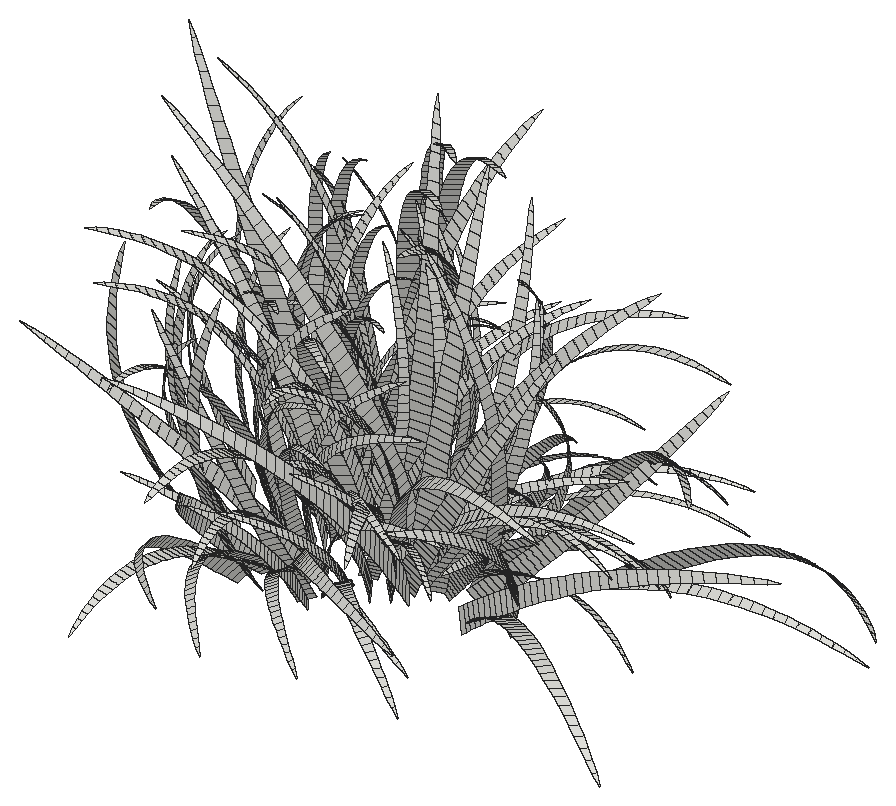
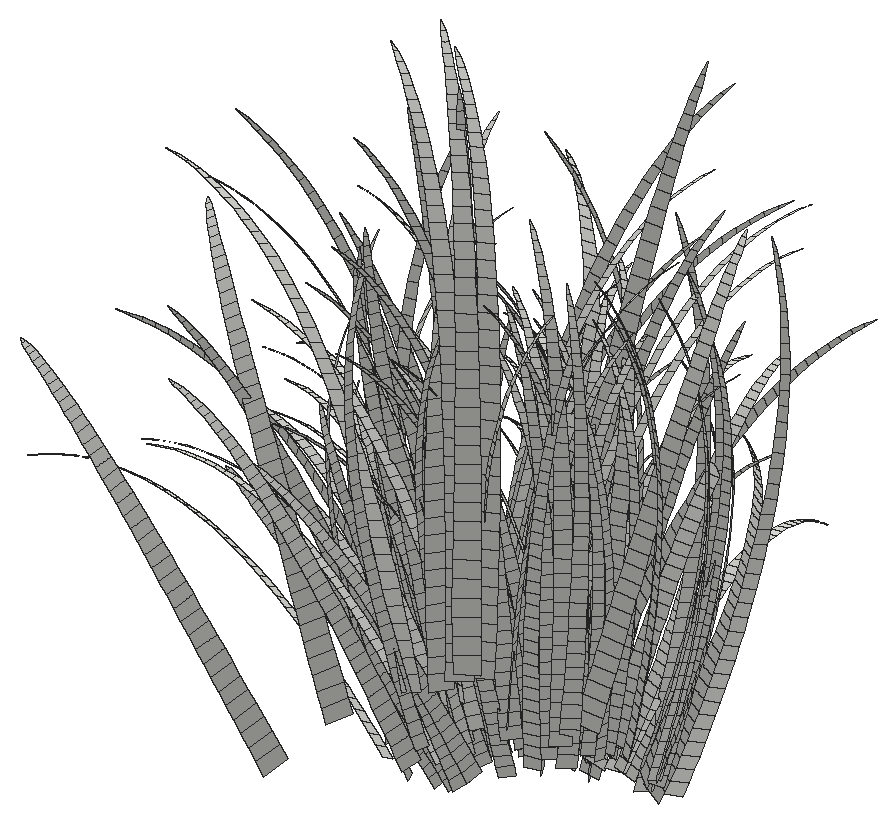
# SketchUp Ruby script. Lengths in inches.
U = 1.inch
M = Sketchup.active_model
def pt(a) = Geom::Point3d.new(a.map { |v| v * U })
def face(e, loops, mat)
  f = e.add_face(loops[0].map { |a| pt(a) })
  loops[1..].each { |l| e.add_face(l.map { |a| pt(a) }).erase! }
  f.material = f.back_material = mat if mat
  f
end
# faces: each face lists its corners as indices into pts; further lists are holes
def faces(e, pts, list, mat = nil) = list.each { |f| face(e, (f[0].is_a?(Array) ? f : [f]).map { |l| l.map { |i| pts[i] } }, mat) }
# xy, xz, yz: faces in a plane at the given z, y or x. An outline is a flat list of corners, or four numbers for a rectangle; further outlines are holes
def ring(l) = l.size == 4 ? [[l[0], l[1]], [l[2], l[1]], [l[2], l[3]], [l[0], l[3]]] : l.each_slice(2).to_a
def flat(e, list, mat, &to3) = list.each { |f| face(e, (f[0].is_a?(Array) ? f : [f]).map { |l| ring(l).map { |u, v| to3.(u, v) } }, mat) }
def xy(e, z, list, mat = nil) = flat(e, list, mat) { |x, y| [x, y, z] }
def xz(e, y, list, mat = nil) = flat(e, list, mat) { |x, z| [x, y, z] }
def yz(e, x, list, mat = nil) = flat(e, list, mat) { |y, z| [x, y, z] }
def lines(e, pts, list) = list.each { |a, b| e.add_line(pt(pts[a]), pt(pts[b])) }
# prism: a flat outline (further loops are holes) pulled along v
def prism(e, loops, v, mat = nil)
  f = face(e, loops, mat); d = Geom::Vector3d.new(v.map { |x| x * U })
  f.pushpull(f.normal.samedirection?(d) ? d.length : -d.length)
end
def box(e, o, s, mat = nil) = prism(e, [[o, [o[0] + s[0], o[1], o[2]], [o[0] + s[0], o[1] + s[1], o[2]], [o[0], o[1] + s[1], o[2]]]], [0, 0, s[2]], mat)
def at(x, y, z, deg = 0) = Geom::Transformation.translation(pt([x, y, z])) * Geom::Transformation.rotation(ORIGIN, Z_AXIS, deg.degrees)
def axes(o, x, y, z) = Geom::Transformation.new([*x, 0, *y, 0, *z, 0, *pt(o).to_a, 1])
def part(name) = M.definitions.add(name)
# library, detail: a bought-in or finely detailed component or shape, given as its bounding box
def library(name, o, s) = part(name).tap { |d| box(d.entities, o, s) }
def detail(e, o, s) = box(e.add_group.entities, o, s)
def put(e, d, t, mat = nil) = e.add_instance(d, t).tap { |i| i.material = mat if mat }
def group(e, t, mat = nil) = e.add_group.tap { |g| g.transformation = t; g.material = mat if mat }.entities
root = M.entities
c1 = part("fur_instance\#8")
p = [[-0.25,1.49,0.03],[0.25,-1.49,-0.03],[0.44,-1.47,1.51],[-0.05,1.47,1.57],[0.65,-1.44,3.05],[0.16,1.45,3.11],
  [0.86,-1.42,4.59],[0.38,1.44,4.65],[1.1,-1.39,6.13],[0.62,1.43,6.18],[1.34,-1.35,7.66],[0.875,1.42,7.72],
  [1.6,-1.32,9.19],[1.14,1.41,9.25],[1.88,-1.28,10.72],[1.43,1.41,10.78],[2.18,-1.24,12.25],[1.73,1.41,12.3],
  [2.49,-1.19,13.77],[2.05,1.41,13.82],[2.83,-1.15,15.29],[2.4,1.41,15.34],[3.18,-1.09,16.8],[2.76,1.42,16.85],
  [3.56,-1.03,18.31],[3.14,1.43,18.35],[3.96,-0.97,19.81],[3.55,1.44,19.85],[4.38,-0.91,21.3],[3.99,1.46,21.35],
  [4.84,-0.83,22.78],[4.45,1.48,22.83],[5.32,-0.76,24.26],[4.93,1.51,24.31],[5.82,-0.67,25.73],[5.45,1.54,25.77],
  [6.36,-0.59,27.18],[6,1.57,27.23],[6.93,-0.49,28.625],[6.58,1.61,28.67],[7.54,-0.39,30.05],[7.19,1.66,30.1],
  [8.18,-0.28,31.47],[7.84,1.71,31.51],[8.85,-0.16,32.86],[8.53,1.77,32.9],[9.57,-0.04,34.24],[9.25,1.83,34.27],
  [10.32,0.09,35.59],[10.02,1.9,35.625],[11.12,0.23,36.92],[10.82,1.97,36.95],[11.95,0.38,38.22],[11.67,2.06,38.25],
  [12.84,0.54,39.49],[12.57,2.14,39.52],[13.76,0.71,40.73],[13.51,2.24,40.76],[14.73,0.89,41.93],[14.49,2.34,41.95],
  [15.75,1.08,43.09],[15.52,2.45,43.11],[16.82,1.28,44.2],[16.6,2.5625,44.23],[17.93,1.5,45.27],[17.73,2.68,45.29],
  [19.08,1.73,46.28],[18.9,2.81,46.3],[20.29,1.97,47.24],[20.125,2.93,47.26],[21.53,2.22,48.13],[21.39,3.0625,48.15],
  [22.82,2.5,48.96],[22.7,3.1875,48.98],[24.14,2.8125,49.72],[24.06,3.3,49.73],[25.48,3.27,50.41]]
faces(c1.entities,p,[[0,1,2,3],[3,2,4,5],[5,4,6,7],[7,6,8,9],[9,8,10,11],[11,10,12,13],[13,12,14,15],[15,14,16,17],
  [17,16,18,19],[19,18,20,21],[21,20,22,23],[23,22,24,25],[25,24,26,27],[27,26,28,29],[29,28,30,31],[31,30,32,33],
  [33,32,34,35],[35,34,36,37],[37,36,38,39],[39,38,40,41],[41,40,42,43],[43,42,44,45],[45,44,46,47],[47,46,48,49],
  [49,48,50,51],[51,50,52,53],[53,52,54,55],[55,54,56,57],[57,56,58,59],[59,58,60,61],[61,60,62,63],[63,62,64,65],
  [65,64,66,67],[67,66,68,69],[69,68,70,71],[71,70,72,73],[73,72,74,75],[75,74,76]])
put(root,c1,axes([297.34,24.49,10.07],[0.22754,0.09548,0.30287],[-0.3741,0.10321,0.18489],[-0.01658,-0.28689,0.27555]))
put(root,c1,axes([298.36,29.48,15.33],[0.08571,-0.27266,-0.13744],[0.42739,0.02102,0.03088],[-0.01459,-0.16231,0.42441]))
put(root,c1,axes([298.25,24.62,10.32],[0.14483,0.12085,0.20815],[-0.30882,0.08881,0.09603],[-0.01291,-0.19862,0.26445]))
put(root,c1,axes([297.38,27.93,13.53],[0.30966,0.098,0.10011],[-0.20983,0.22175,0.06913],[-0.05457,-0.13112,0.36799]))
put(root,c1,axes([297.55,26.52,12.34],[0.32914,-0.02019,0.08794],[-0.06155,0.19695,0.14966],[-0.07419,-0.15278,0.30582]))
put(root,c1,axes([302.33,24.8,10.55],[-0.40749,-0.00335,0.18025],[-0.12021,-0.15441,-0.30655],[0.11437,-0.28118,0.27754]))
put(root,c1,axes([299.27,26.41,12.88],[-0.00998,-0.21329,-0.19726],[0.39469,-0.01957,-0.03476],[0.02221,-0.19303,0.35251]))
put(root,c1,axes([297.15,25.85,11.82],[0.33918,0.02077,0.08926],[-0.11622,0.19982,0.16012],[-0.0464,-0.17067,0.32217]))
put(root,c1,axes([302.64,29.66,13.99],[-0.38125,-0.04643,0.1073],[0.06668,-0.27303,-0.05684],[0.10363,-0.09301,0.39245]))
put(root,c1,axes([302.09,25.9375,11.41],[-0.30784,-0.04638,0.08341],[0.04021,-0.18889,-0.13984],[0.09826,-0.13618,0.29147]))
put(root,c1,axes([297.93,24.99,10.86],[0.34312,-0.02724,0.07631],[-0.06105,0.16155,0.2245],[-0.05704,-0.19865,0.27364]))
put(root,c1,axes([298.34,24.67,10.57],[0.25415,0.10614,0.20022],[-0.29634,0.1349,0.16955],[-0.01477,-0.22734,0.30268]))
put(root,c1,axes([302.43,27.59,14.25],[-0.34392,-0.19747,-0.05942],[0.31246,-0.1879,-0.23256],[0.10907,-0.21637,0.42646]))
put(root,c1,axes([298.55,30.67,13.78],[0.22131,-0.22629,0.02615],[0.29382,0.13921,-0.0109],[-0.01591,-0.03849,0.37643]))
put(root,c1,axes([300.79,24.4,10.07],[-0.08897,-0.12733,-0.31327],[0.39814,-0.02359,-0.11091],[0.04663,-0.26995,0.25847]))
put(root,c1,axes([301.35,29.07,12.71],[-0.18067,-0.19345,0.07522],[0.26975,-0.14432,-0.061],[0.08262,-0.03764,0.32955]))
put(root,c1,axes([302.4375,26.68,13.18],[-0.30501,-0.19584,-0.06885],[0.3125,-0.16513,-0.21481],[0.1025,-0.20334,0.40077]))
put(root,c1,axes([300.66,30.47,12.875],[-0.05382,-0.24378,0.08465],[0.33677,-0.06068,-0.04502],[0.04922,-0.00382,0.34004]))
put(root,c1,axes([298.89,26.04,12.12],[0.26522,0.09384,0.11083],[-0.21458,0.15991,0.13303],[-0.0124,-0.16608,0.30419]))
put(root,c1,axes([302.32,24.36,9.24],[-0.2996,-0.07248,0.07639],[0.02633,-0.11445,-0.25289],[0.12958,-0.19663,0.20724]))
put(root,c1,axes([302.84,26.03,12.1],[-0.30808,0.0964,0.26106],[-0.2636,-0.1875,-0.11584],[0.13613,-0.2298,0.33276]))
put(root,c1,axes([302.32,24.34,9.32],[-0.1838,0.08779,0.29069],[-0.31205,-0.09811,-0.08599],[0.09749,-0.23969,0.23659]))
put(root,c1,axes([298.55,28.32,13.11],[0.33703,-0.0606,0.00869],[0.04934,0.22775,0.04178],[-0.02278,-0.08013,0.34741]))
put(root,c1,axes([301.15,28.07,12.85],[-0.08647,-0.22321,-0.0256],[0.3195,-0.05984,-0.10171],[0.08204,-0.09177,0.33353]))
put(root,c1,axes([298.93,24.11,9.43],[0.31431,-0.11382,-0.22646],[0.27893,0.07249,0.25434],[-0.01591,-0.27534,0.26445]))
put(root,c1,axes([299.05,27.16,12.77],[0.30618,-0.11178,-0.04367],[0.14225,0.17991,0.09998],[-0.0113,-0.12571,0.32871]))
put(root,c1,axes([302.84,28.1,12.3],[-0.3018,-0.05533,0.14889],[0.04839,-0.22497,-0.0736],[0.14879,-0.08814,0.30643]))
put(root,c1,axes([298.8,28.85,13.53],[0.33228,-0.11223,-0.01481],[0.12989,0.21816,0.04248],[-0.01045,-0.08682,0.36317]))
put(root,c1,axes([298.86,30.74,14.82],[0.2513,-0.23591,-0.02705],[0.31438,0.16202,-0.0286],[0.02842,-0.06817,0.4118]))
put(root,c1,axes([303.34,26.51,13.1875],[-0.20765,0.20524,0.34836],[-0.46933,-0.12275,-0.04529],[0.10847,-0.29849,0.40724]))
put(root,c1,axes([299.4375,24.06,9.36],[0.23528,0.12192,0.28082],[-0.37572,0.07027,0.22703],[0.05067,-0.29334,0.28087]))
put(root,c1,axes([302.89,29.79,12.49],[-0.26364,-0.1277,0.16127],[0.17439,-0.21809,-0.03735],[0.14552,-0.02258,0.31606]))
put(root,c1,axes([299.78,27.4375,13.63],[0.21857,-0.21363,-0.1219],[0.32632,0.12674,0.03328],[0.03098,-0.14429,0.38367]))
put(root,c1,axes([302.0625,26.01,12.41],[-0.08548,-0.19985,-0.26017],[0.42158,-0.01554,-0.13787],[0.09092,-0.25018,0.34134]))
put(root,c1,axes([299.15,24.38,10.15],[0.39204,-0.05893,-0.06456],[0.07903,0.1141,0.3176],[-0.01514,-0.26203,0.25167]))
put(root,c1,axes([300.34,27.34,13.09],[0.20316,0.18695,0.05206],[-0.29596,0.1361,0.10285],[0.04697,-0.12733,0.35285]))
put(root,c1,axes([300.29,29.89,13.24],[0.241,-0.19394,-0.00595],[0.25165,0.15803,-0.0286],[0.01565,-0.04576,0.35642]))
put(root,c1,axes([300.23,24.37,10.06],[0.20909,-0.10864,-0.30363],[0.35015,0.0704,0.13483],[0.04661,-0.26986,0.25839]))
put(root,c1,axes([302.13,24.96,10.65],[0.0034,-0.17259,-0.2459],[0.3736,0.02284,-0.07022],[0.07897,-0.21729,0.29647]))
put(root,c1,axes([304.83,28.53,14.14],[-0.33019,-0.21589,-0.02043],[0.30998,-0.1841,-0.23665],[0.14334,-0.19866,0.4252]))
put(root,c1,axes([306.23,27.17,12.88],[-0.44601,0.0603,0.27836],[-0.22496,-0.25265,-0.21525],[0.16772,-0.28312,0.40997]))
put(root,c1,axes([300.14,25.48,11.52],[0.31524,-0.06334,-0.07199],[0.09612,0.1672,0.15091],[0.01854,-0.16113,0.29426]))
put(root,c1,axes([305.13,26.27,11.21],[-0.38378,-0.04877,0.18024],[-0.02944,-0.22334,-0.21648],[0.17648,-0.20752,0.33035]))
put(root,c1,axes([301.71,27.32,12.9],[0.09016,-0.23072,-0.1049],[0.34864,0.05757,-0.04796],[0.06396,-0.12072,0.35681]))
put(root,c1,axes([300.71,28.48,12.82],[0.28641,-0.13175,-0.03296],[0.16621,0.19382,-0.00842],[0.02384,-0.06063,0.3387]))
put(root,c1,axes([304.25,25.28,9.26],[-0.26262,-0.12182,0.05251],[0.09128,-0.10048,-0.25575],[0.16729,-0.17618,0.20619]))
put(root,c1,axes([304.83,25.73,9.93],[-0.30829,-0.09539,0.14082],[0.00903,-0.14692,-0.25308],[0.18557,-0.19544,0.22873]))
put(root,c1,axes([302.31,30.2,11.78],[0.03803,-0.23615,0.09237],[0.30529,0.00187,-0.1209],[0.10385,0.01684,0.29612]))
put(root,c1,axes([303.54,26.1875,10.96],[-0.17541,-0.18465,-0.02445],[0.23008,-0.0678,-0.21965],[0.16634,-0.14325,0.26122]))
put(root,c1,axes([301.04,25.375,11.33],[0.25986,-0.11185,-0.13998],[0.20362,0.14616,0.09388],[0.04858,-0.15915,0.29774]))
put(root,c1,axes([300.67,28.46,13.55],[0.22798,-0.18767,-0.11254],[0.27671,0.15509,-0.02037],[0.07789,-0.11087,0.35837]))
put(root,c1,axes([306.9,25.87,10.72],[-0.48988,-0.11693,0.12815],[0.03908,-0.18796,-0.41221],[0.21173,-0.3213,0.33863]))
put(root,c1,axes([304.08,26.78,11.13],[-0.20056,0.10644,0.21815],[-0.1976,-0.18803,0.05052],[0.19039,-0.12136,0.26701]))
put(root,c1,axes([303.36,27.03,12.83],[-0.04495,-0.24966,-0.14848],[0.39596,-0.00054,-0.1471],[0.12613,-0.17481,0.37414]))
put(root,c1,axes([300.875,28.02,12.78],[0.31334,0.05722,-0.07403],[-0.08122,0.21863,0.071],[0.08023,-0.08975,0.32618]))
put(root,c1,axes([304.8,27.75,10.98],[-0.23233,0.07819,0.21635],[-0.13938,-0.21462,0.04879],[0.20297,-0.09356,0.26698]))
put(root,c1,axes([302.16,30.1,13.69],[0.15425,-0.25107,-0.03735],[0.33478,0.10551,-0.10575],[0.09996,-0.05813,0.37518]))
put(root,c1,axes([304.91,27.45,12.12],[-0.25388,-0.20378,0.01616],[0.23529,-0.11773,-0.26393],[0.19902,-0.17138,0.31253]))
put(root,c1,axes([301.81,24.55,10.08],[0.19971,-0.08632,-0.29459],[0.31288,0.10372,0.09875],[0.09992,-0.24566,0.24248]))
put(root,c1,axes([305.41,29.01,11.21],[-0.27508,0.01899,0.22955],[-0.04819,-0.2486,0.02313],[0.21789,-0.06738,0.28047]))
put(root,c1,axes([301.65,28.92,12.46],[0.28163,-0.12087,-0.06722],[0.14848,0.20348,-0.06709],[0.08102,-0.03691,0.32316]))
put(root,c1,axes([300.74,25.01,11.39],[0.45568,0.06765,0.06956],[-0.16773,0.20168,0.31955],[0.04218,-0.28469,0.37786]))
put(root,c1,axes([301.56,25.46,11.47],[0.33477,0.08293,0.02574],[-0.13812,0.14697,0.24654],[0.07654,-0.21062,0.28736]))
put(root,c1,axes([301.31,28.87,13.17],[0.30114,-0.11966,-0.09813],[0.15874,0.2176,-0.03834],[0.09385,-0.06803,0.34638]))
put(root,c1,axes([305.74,28.81,11.7],[-0.28867,0.02967,0.24792],[-0.09166,-0.25361,-0.00275],[0.22689,-0.10459,0.29846]))
put(root,c1,axes([305.46,26.23,9.98],[-0.26784,-0.15803,0.10336],[0.1003,-0.12666,-0.27197],[0.22305,-0.17007,0.23161]))
put(root,c1,axes([302.53,28.71,12.53],[0.22312,-0.17996,-0.07706],[0.24279,0.15961,-0.06691],[0.09091,-0.0659,0.33552]))
put(root,c1,axes([302.11,27.35,14.32],[0.30189,-0.2143,-0.23607],[0.3879,0.17076,0.0851],[0.07233,-0.23695,0.44329]))
put(root,c1,axes([306.3,29.18,11.54],[-0.3066,-0.07009,0.23185],[0.02539,-0.24972,-0.09835],[0.23047,-0.10624,0.30316]))
put(root,c1,axes([302.74,27.47,12.35],[0.21694,0.18488,-0.0402],[-0.23457,0.13588,0.16772],[0.14294,-0.11176,0.31472]))
put(root,c1,axes([306.73,27.34,10.91],[-0.20769,0.14499,0.26631],[-0.28732,-0.19256,0.04919],[0.20383,-0.17553,0.32009]))
put(root,c1,axes([305.49,27.83,13.38],[-0.08102,0.22851,0.2885],[-0.42602,-0.11882,0.13225],[0.19883,-0.2338,0.37219]))
put(root,c1,axes([301.94,25.29,11.29],[0.40091,0.03016,-0.06734],[-0.01586,0.18451,0.26625],[0.0848,-0.23335,0.31837]))
put(root,c1,axes([302.89,32.5,17.82],[0.25572,-0.30691,-0.1555],[0.45234,0.17411,-0.05741],[0.11289,-0.16068,0.51939]))
put(root,c1,axes([303.53,28.55,14.42],[0.21342,0.25446,0.08921],[-0.38491,0.1062,0.2129],[0.1393,-0.19307,0.41321]))
put(root,c1,axes([303.13,24.86,9.67],[0.22226,-0.03579,-0.23917],[0.20428,0.13118,0.1145],[0.13006,-0.19737,0.20802]))
put(root,c1,axes([302.86,26.07,11.88],[0.25415,-0.10802,-0.25116],[0.27378,0.16143,0.07847],[0.12542,-0.21172,0.30658]))
put(root,c1,axes([305.11,31.45,15.75],[-0.0769,-0.31872,-0.07944],[0.43795,-0.01955,-0.2265],[0.19894,-0.15553,0.43799]))
put(root,c1,axes([303.3,30.9375,16.79],[0.29435,-0.27412,-0.16204],[0.41262,0.19204,-0.0101],[0.09002,-0.16992,0.50222]))
put(root,c1,axes([302.8,24.9,10.11],[0.31893,0.00084,-0.14381],[0.07397,0.17023,0.18028],[0.10993,-0.18556,0.2687]))
put(root,c1,axes([303.4375,27.83,13.15],[0.22284,0.22267,0.01676],[-0.30608,0.12329,0.20104],[0.14725,-0.15151,0.36439]))
put(root,c1,axes([304.81,26.24,11.52],[0.02363,-0.22016,-0.24514],[0.39411,0.08072,-0.15296],[0.18102,-0.21286,0.33886]))
put(root,c1,axes([304.35,26.14,10.36],[0.11227,-0.15154,-0.20337],[0.26794,0.12668,-0.08881],[0.16703,-0.14384,0.2623]))
put(root,c1,axes([303.07,32.69,17.52],[0.32353,-0.26537,-0.15942],[0.39128,0.2201,-0.02856],[0.1103,-0.157,0.50748]))
put(root,c1,axes([306.99,28.03,11.25],[-0.12843,0.20843,0.21843],[-0.31581,-0.15815,0.16065],[0.23054,-0.14695,0.32332]))
put(root,c1,axes([306.27,31.36,12.34],[-0.13308,-0.26326,0.14802],[0.2903,-0.12144,-0.21379],[0.24345,-0.04095,0.31921]))
put(root,c1,axes([302.52,24.75,10.52],[0.40095,-0.04465,-0.28976],[0.25669,0.16722,0.27357],[0.12816,-0.31508,0.31101]))
put(root,c1,axes([303.85,24.95,10.14],[0.21212,-0.09265,-0.34742],[0.34111,0.15542,0.06154],[0.17306,-0.26262,0.27679]))
put(root,c1,axes([304.53,27.53,12.17],[0.27009,0.18151,-0.02583],[-0.2385,0.16041,0.19025],[0.14014,-0.14419,0.34679]))
put(root,c1,axes([305.1,30.01,10.22],[0.09946,-0.22813,0.00742],[0.24835,0.06793,-0.21012],[0.1872,-0.00489,0.26052]))
put(root,c1,axes([306.85,26.9,11.58],[-0.00683,0.24532,0.26139],[-0.4333,-0.07786,0.1796],[0.19869,-0.23364,0.37193]))
put(root,c1,axes([305.04,28.56,10.66],[0.10211,-0.20387,-0.09855],[0.23938,0.11146,-0.19109],[0.20305,-0.06279,0.26137]))
put(root,c1,axes([306.16,28.95,9.54],[-0.06535,-0.22674,0.13107],[0.20945,-0.07623,-0.22504],[0.24597,-0.02324,0.21537]))
put(root,c1,axes([306.87,27.41,10.26],[-0.11302,0.153,0.26635],[-0.25481,-0.18419,0.15446],[0.26582,-0.14677,0.2473]))
put(root,c1,axes([307.28,27.4,10.09],[-0.13627,0.14133,0.28477],[-0.25117,-0.20069,0.13612],[0.2725,-0.15046,0.25352]))
put(root,c1,axes([304.38,29.98,10.89],[0.23395,-0.13822,-0.12541],[0.13453,0.19634,-0.17104],[0.18884,-0.00494,0.2628]))
put(root,c1,axes([309.19,28.14,11.03],[-0.30608,0.01652,0.36552],[-0.2093,-0.26205,-0.09314],[0.28918,-0.22048,0.30027]))
put(root,c1,axes([304.77,26.93,10.57],[0.25146,0.13747,-0.12144],[-0.11784,0.16285,0.18448],[0.18778,-0.1197,0.26336]))
put(root,c1,axes([307.41,27.625,10.17],[-0.13638,-0.24622,-0.04178],[0.25232,-0.00872,-0.31404],[0.27351,-0.15102,0.25446]))
put(root,c1,axes([307.96,30.11,9.72],[-0.18802,-0.2009,0.2136],[0.15844,-0.17448,-0.20851],[0.28488,-0.06696,0.24446]))
put(root,c1,axes([306.29,26.3,10.49],[0.15586,0.20567,0.19062],[-0.32905,-0.02152,0.28384],[0.21907,-0.23072,0.27002]))
put(root,c1,axes([305.04,28.98,12.72],[0.33777,-0.06805,-0.19427],[0.11791,0.26248,-0.00695],[0.17416,-0.10316,0.35867]))
put(root,c1,axes([305.88,29.36,9.75],[0.12899,-0.19626,-0.10232],[0.17724,0.13637,-0.23923],[0.24574,-0.02322,0.21517]))
put(root,c1,axes([305.42,27.18,10.76],[0.29043,0.0064,-0.22579],[0.06951,0.22909,0.0737],[0.20194,-0.12872,0.28321]))
put(root,c1,axes([305.96,28.06,11.31],[0.24712,-0.0965,-0.24934],[0.19671,0.22236,-0.03054],[0.21358,-0.13615,0.29954]))
put(root,c1,axes([305.7,26.87,10.97],[0.33871,0.04215,-0.20809],[0.0397,0.228,0.15673],[0.19608,-0.16885,0.30791]))
put(root,c1,axes([310.91,27.67,9.69],[-0.32027,-0.26261,0.03115],[0.24097,-0.10763,-0.40652],[0.31258,-0.23832,0.32457]))
put(root,c1,axes([306.65,29.41,9.66],[0.13998,-0.20119,-0.1139],[0.18152,0.14824,-0.24709],[0.25697,-0.02428,0.225]))
put(root,c1,axes([305.51,29.47,14.17],[0.42752,0.07803,-0.15016],[-0.06383,0.27992,0.17466],[0.16812,-0.17298,0.41603]))
put(root,c1,axes([305.98,29.04,11.375],[0.28212,0.09572,-0.22762],[-0.08022,0.24373,0.08309],[0.22884,-0.07077,0.29456]))
put(root,c1,axes([306.72,28.14,10.05],[0.14119,-0.14163,-0.23922],[0.19799,0.1965,-0.1586],[0.26602,-0.10193,0.23276]))
put(root,c1,axes([305.74,26.48,12.09],[0.42799,-0.0644,-0.27533],[0.2288,0.24399,0.20262],[0.16294,-0.27505,0.39829]))
put(root,c1,axes([306.82,28.16,10.57],[0.24831,-0.10238,-0.23706],[0.17169,0.23302,-0.06981],[0.22616,-0.10425,0.29749]))
put(root,c1,axes([306.53,29.74,10.82],[0.28927,0.00402,-0.23977],[0.02368,0.25909,-0.00208],[0.22645,-0.07003,0.29149]))
put(root,c1,axes([307.02,31.21,11.13],[0.23822,-0.17838,-0.16309],[0.19592,0.21585,-0.19099],[0.23514,-0.03955,0.30831]))
put(root,c1,axes([307.17,27.27,12.13],[0.32533,0.2365,0.05188],[-0.31811,0.13076,0.32893],[0.20862,-0.24531,0.39052]))
put(root,c1,axes([308.75,28.38,9.72],[0.09146,0.2529,0.10201],[-0.28326,-0.03766,0.31256],[0.28385,-0.15672,0.26408]))
put(root,c1,axes([307.4375,30.66,14.51],[0.41841,-0.08805,-0.24207],[0.17069,0.31234,0.03012],[0.20217,-0.15807,0.44512]))
put(root,c1,axes([310.07,27,9.6875],[0.214,-0.12431,-0.41458],[0.3864,0.21791,-0.01296],[0.26577,-0.2799,0.32758]))
put(root,c1,axes([310.85,31.57,12.3125],[0.10249,-0.29776,-0.17699],[0.37955,0.14559,-0.26879],[0.29452,-0.13576,0.38741]))
put(root,c1,axes([309.01,26.92,9.41],[0.34459,0.19403,-0.14464],[-0.11378,0.16849,0.33964],[0.28302,-0.21579,0.29387]))
put(root,c1,axes([309.77,29.43,9.78],[0.28699,0.07592,-0.32341],[0.01679,0.27611,0.10267],[0.31448,-0.1205,0.27516]))
put(root,c1,axes([312.89,33.58,10.01],[0.14997,-0.26821,-0.20593],[0.27436,0.20632,-0.3189],[0.36228,-0.08516,0.31088]))
